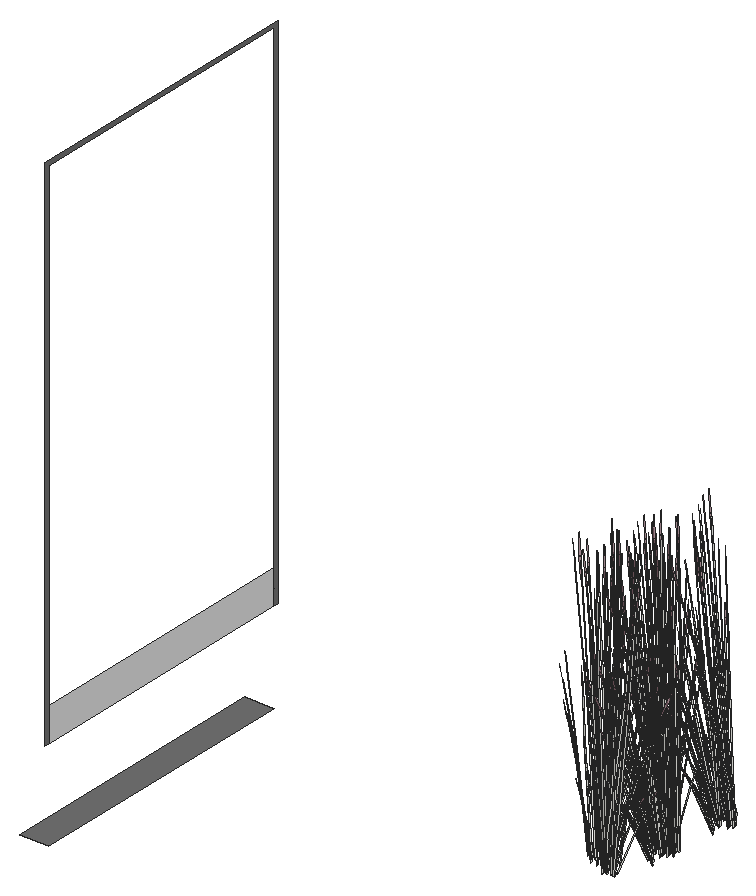
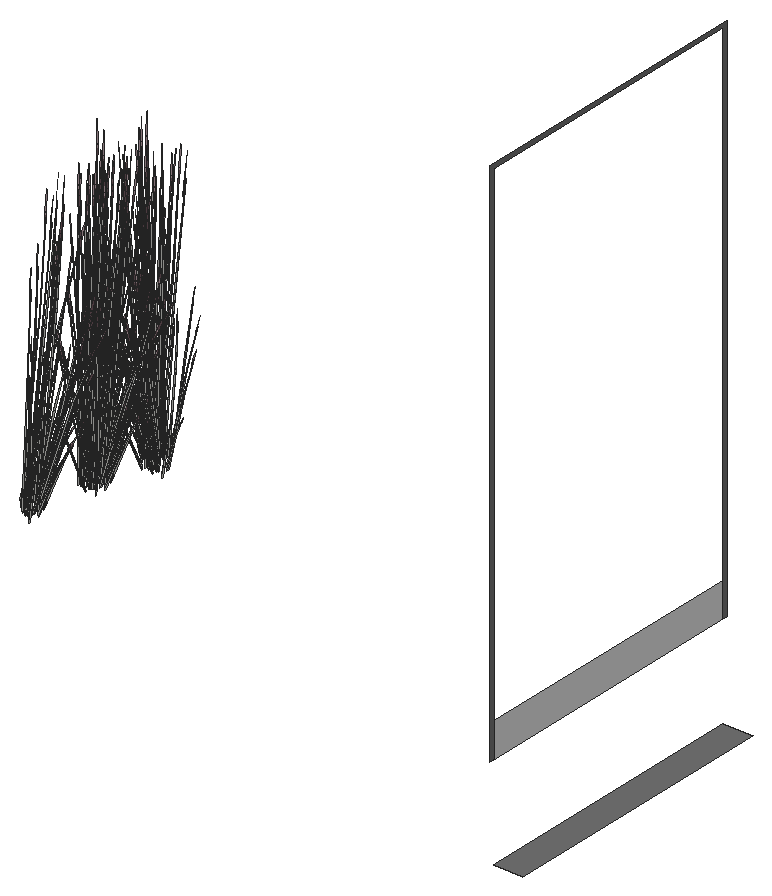
# SketchUp Ruby script. Lengths in inches.
U = 1.inch
M = Sketchup.active_model
def pt(a) = Geom::Point3d.new(a.map { |v| v * U })
def face(e, loops, mat)
  f = e.add_face(loops[0].map { |a| pt(a) })
  loops[1..].each { |l| e.add_face(l.map { |a| pt(a) }).erase! }
  f.material = f.back_material = mat if mat
  f
end
# faces: each face lists its corners as indices into pts; further lists are holes
def faces(e, pts, list, mat = nil) = list.each { |f| face(e, (f[0].is_a?(Array) ? f : [f]).map { |l| l.map { |i| pts[i] } }, mat) }
# xy, xz, yz: faces in a plane at the given z, y or x. An outline is a flat list of corners, or four numbers for a rectangle; further outlines are holes
def ring(l) = l.size == 4 ? [[l[0], l[1]], [l[2], l[1]], [l[2], l[3]], [l[0], l[3]]] : l.each_slice(2).to_a
def flat(e, list, mat, &to3) = list.each { |f| face(e, (f[0].is_a?(Array) ? f : [f]).map { |l| ring(l).map { |u, v| to3.(u, v) } }, mat) }
def xy(e, z, list, mat = nil) = flat(e, list, mat) { |x, y| [x, y, z] }
def xz(e, y, list, mat = nil) = flat(e, list, mat) { |x, z| [x, y, z] }
def yz(e, x, list, mat = nil) = flat(e, list, mat) { |y, z| [x, y, z] }
def lines(e, pts, list) = list.each { |a, b| e.add_line(pt(pts[a]), pt(pts[b])) }
# prism: a flat outline (further loops are holes) pulled along v
def prism(e, loops, v, mat = nil)
  f = face(e, loops, mat); d = Geom::Vector3d.new(v.map { |x| x * U })
  f.pushpull(f.normal.samedirection?(d) ? d.length : -d.length)
end
def box(e, o, s, mat = nil) = prism(e, [[o, [o[0] + s[0], o[1], o[2]], [o[0] + s[0], o[1] + s[1], o[2]], [o[0], o[1] + s[1], o[2]]]], [0, 0, s[2]], mat)
def at(x, y, z, deg = 0) = Geom::Transformation.translation(pt([x, y, z])) * Geom::Transformation.rotation(ORIGIN, Z_AXIS, deg.degrees)
def axes(o, x, y, z) = Geom::Transformation.new([*x, 0, *y, 0, *z, 0, *pt(o).to_a, 1])
def part(name) = M.definitions.add(name)
# library, detail: a bought-in or finely detailed component or shape, given as its bounding box
def library(name, o, s) = part(name).tap { |d| box(d.entities, o, s) }
def detail(e, o, s) = box(e.add_group.entities, o, s)
def put(e, d, t, mat = nil) = e.add_instance(d, t).tap { |i| i.material = mat if mat }
def group(e, t, mat = nil) = e.add_group.tap { |g| g.transformation = t; g.material = mat if mat }.entities
root = M.entities
M.materials.add("LightPink_Translucent").color = [144, 107, 117]
M.materials["LightPink_Translucent"].alpha = 0.75
M.materials.add("M01_Silver_Fog").color = [224, 224, 224]
M.materials.add("M06_Steel_Smoke").color = [114, 114, 114]
c1 = part("blade")
p = [[2.15,0.21,22],[0,0.17,0],[0.09,0.45,0],[2.18,0.31,22],[2.29,0.31,22],[0.38,0.45,0],
  [2.48,0.24,33],[2.49,0.24,33],[2.48,0.22,33]]
faces(c1.entities,p,[[0,1,2,3],[4,5,2,3],[6,3,4,7],[8,0,3,6]])
c2 = part("seeds")
p = [[0.3,-0.1,1.38],[-0.01,-0.03,1.59],[-0.01,-0.03,0.03],[0.14,-0.07,-0.07],[0.29,-0.03,3],[0.15,0.01,3.11]]
faces(c2.entities,p,[[0,1,2,3],[1,0,4,5]],"LightPink_Translucent")
c3 = part("blade with seeds")
put(c3.entities,c1,at(0,0,0))
put(c3.entities,c2,axes([2.4,0.25,30.99],[1.5799,-0.05474,1.17369],[-0.12525,1.92788,0.29478],[-0.07173,-0.02425,1.56792]))
xy(root,503,[[204,295,210,353]],"M06_Steel_Smoke")
yz(root,210,[[295,522,353,529]],"M01_Silver_Fog")
yz(root,210,[[294,522,295,522,295,629,353,629,353,522,354,522,354,630,294,630]],"M06_Steel_Smoke")
put(root,c3,axes([306.14,314.57,525.875],[0.17434,-0.11391,1.71376],[0.14677,0.52637,0.13857],[-0.27369,0.11897,0.73262]))
put(root,c3,axes([305.6,315.47,524.59],[0.17462,0.04421,1.43002],[0.11254,0.45156,-0.30754],[-0.23719,0.08453,0.61141]))
put(root,c3,axes([306.16,314.32,526.68],[-0.13612,0.48987,-0.51099],[-0.46669,-0.16791,-0.3958],[-0.1879,0.04492,0.97773]))
put(root,c3,axes([305.23,316.41,524.77],[0.2094,-0.24408,1.1486],[0.08263,0.38639,0.84392],[-0.15132,0.06919,0.25299]))
put(root,c3,axes([306.78,314.92,525.875],[0.1255,-0.16547,1.71376],[0.31687,0.44665,0.13857],[-0.21734,0.2034,0.73262]))
put(root,c3,axes([306.02,315.36,526.53],[-0.43736,0.07697,-0.35414],[-0.11549,-0.43998,0.4572],[-0.12533,0.11818,0.87481]))
put(root,c3,axes([305.79,316.66,523.49],[0.0674,0.0538,1.76342],[0.11428,0.49852,-0.26939],[-0.14937,0.10631,0.30037]))
put(root,c3,axes([306.6875,315.33,525.875],[0.09355,-0.18511,1.71376],[0.39247,0.38307,0.13857],[-0.17705,0.23875,0.73262]))
put(root,c3,axes([306.38,315.41,526.68],[0.12908,0.49174,-0.51099],[-0.48882,0.08602,-0.3958],[-0.14008,0.13208,0.97773]))
put(root,c3,axes([307.2,316.41,524.375],[-0.31414,0.53965,0],[-0.52557,-0.30095,-0.51607],[-0.1197,-0.06854,1.63711]))
put(root,c3,axes([306.63,317.19,524.59],[0.15856,-0.08496,1.43002],[0.39147,0.25616,-0.30754],[-0.11652,0.22165,0.61141]))
put(root,c3,axes([306.79,316.375,526.53],[-0.33997,0.28354,-0.35414],[-0.32182,-0.32376,0.4572],[-0.04897,0.1645,0.87481]))
put(root,c3,axes([308.53,315.53,524.06],[-0.33843,0.40479,-0.62353],[-0.42041,-0.36705,-0.16365],[-0.13561,0.10098,1.37633]))
put(root,c3,axes([310.75,324.63,525.875],[0.20841,-0.0122,1.71376],[-0.13825,0.52864,0.13857],[-0.297,-0.0327,0.73262]))
put(root,c3,axes([308.77,315.3,524.46],[-0.49063,-0.43346,-0.25192],[0.41285,-0.48673,0.5513],[-0.13212,0.05071,1.68216]))
put(root,c3,axes([307.02,316.08,527.34],[-0.01307,0.49815,-0.7886],[-0.55054,-0.03346,0.09517],[-0.0581,0.21104,1.11556]))
put(root,c3,axes([307.01,317.48,524.77],[-0.013,-0.32022,1.1486],[0.32493,0.22839,0.84392],[-0.0639,0.15263,0.25299]))
put(root,c3,axes([308.52,315.21,524.21],[-0.54562,0.03324,-0.44739],[-0.04934,-0.55185,0.21531],[-0.09768,0.05593,1.43643]))
put(root,c3,axes([307.48,316.13,524.48],[0.47024,0.26927,0.49651],[-0.28107,0.48284,0],[-0.1071,-0.06133,1.57504]))
put(root,c3,axes([310.84,325.56,525.875],[0.17434,-0.11391,1.71376],[0.14677,0.52637,0.13857],[-0.27369,0.11897,0.73262]))
put(root,c3,axes([306.84,316.78,525.36],[0.01104,-0.27801,1.54345],[0.49652,0.14685,0.21329],[-0.04302,0.2963,0.72882]))
put(root,c3,axes([310.29,326.46,524.59],[0.17462,0.04421,1.43002],[0.11254,0.45156,-0.30754],[-0.23719,0.08453,0.61141]))
put(root,c3,axes([309.09,316.63,524.02],[-0.47024,0.26927,-0.49651],[-0.28107,-0.48284,0],[-0.1071,0.06133,1.57504]))
put(root,c3,axes([309.12,316.49,524.19],[-0.31023,-0.54153,-0.05142],[0.52557,-0.30095,0.51607],[-0.12951,0.05156,1.6363]))
put(root,c3,axes([311.84,325.01,525.34],[0.14282,-0.0779,1.77064],[0.04925,0.54394,0.13857],[-0.30935,0.07218,0.63284]))
put(root,c3,axes([307.13,316.24,527],[0.35968,0.36185,-0.5672],[-0.37996,0.3169,-0.43934],[-0.05473,0.18385,1.08528]))
put(root,c3,axes([308.98,316.42,524.03],[-0.46876,-0.13325,-0.30978],[0.11803,-0.46926,0.30978],[-0.0945,0.05411,1.38974]))
put(root,c3,axes([309.25,314.41,524.84],[-0.01373,-0.50706,1.41272],[0.62119,0.13144,0.59816],[-0.14692,0.27746,1.3335]))
put(root,c3,axes([311.375,324.14,526.98],[-0.50227,-0.01297,-0.71045],[0.03373,-0.54602,0.08574],[-0.21278,-0.05762,1.00501]))
put(root,c3,axes([310.97,324.27,524.59],[0.0981,0.14994,1.43002],[-0.22605,0.40756,-0.30754],[-0.23211,-0.09741,0.61141]))
put(root,c3,axes([306.74,316.79,524.82],[0.45645,-0.09537,0.06507],[0.10494,0.38421,-0.86304],[-0.02894,0.19449,0.7736]))
put(root,c3,axes([308.9,315.06,524.67],[0.05855,0.61451,-0.29095],[-0.60981,0.03716,-0.50002],[-0.10738,0.08185,1.59708]))
put(root,c3,axes([310.57,325.08,526.53],[-0.41757,-0.15024,-0.35414],[0.12179,-0.4383,0.4572],[-0.16812,0.04019,0.87481]))
put(root,c3,axes([311.14,323.78,525.875],[0.18664,0.09279,1.71376],[-0.38624,0.38925,0.13857],[-0.24072,-0.1756,0.73262]))
put(root,c3,axes([307.54,315.72,525.875],[-0.0123,-0.2067,1.71376],[0.53301,0.13712,0.13857],[-0.03297,0.29456,0.73262]))
put(root,c3,axes([310.85,325.31,526.68],[-0.13612,0.48987,-0.51099],[-0.46669,-0.16791,-0.3958],[-0.1879,0.04492,0.97773]))
put(root,c3,axes([311.21,324.25,526.68],[-0.36484,0.35674,-0.51099],[-0.31952,-0.37685,-0.3958],[-0.18537,-0.05428,0.97773]))
put(root,c3,axes([310.62,325.28,523.49],[0.01274,0.08487,1.76342],[-0.25688,0.44323,-0.26939],[-0.18246,-0.02234,0.30037]))
put(root,c3,axes([309.93,327.4,524.77],[0.2094,-0.24408,1.1486],[0.08263,0.38639,0.84392],[-0.15132,0.06919,0.25299]))
put(root,c3,axes([308.35,315.94,524.2],[-0.50654,-0.24178,0],[0.24378,-0.50239,0],[0,0,1.62707]))
put(root,c3,axes([309.52,316.55,524.375],[0.31414,0.53965,0],[-0.52557,0.30095,-0.51607],[-0.1197,0.06854,1.63711]))
put(root,c3,axes([311.07,323.91,526.53],[-0.28589,-0.33718,-0.35414],[0.32644,-0.31919,0.4572],[-0.16586,-0.04856,0.87481]))
put(root,c3,axes([311.48,325.91,525.875],[0.1255,-0.16547,1.71376],[0.31687,0.44665,0.13857],[-0.21734,0.2034,0.73262]))
put(root,c3,axes([310.72,326.35,526.53],[-0.43736,0.07697,-0.35414],[-0.11549,-0.43998,0.4572],[-0.12533,0.11818,0.87481]))
put(root,c3,axes([310.48,327.65,523.49],[0.0674,0.0538,1.76342],[0.11428,0.49852,-0.26939],[-0.14937,0.10631,0.30037]))
put(root,c3,axes([309.01,315.18,524.62],[0.37121,0.32357,0.1448],[-0.30963,0.36505,-0.41347],[-0.08619,0.04935,1.26744]))
put(root,c3,axes([310.39,324.72,524.77],[0.32078,-0.03854,1.1486],[-0.20348,0.33954,0.84392],[-0.15852,-0.05093,0.25299]))
put(root,c3,axes([309,314.94,524.72],[0.54562,-0.03324,0.44739],[0.04934,0.55185,-0.21531],[-0.09768,0.05593,1.43643]))
put(root,c3,axes([309.14,316.21,524.33],[0.62903,0.17504,0.30756],[-0.15737,0.62568,-0.36492],[-0.10411,0.07831,1.64885]))
put(root,c3,axes([309.41,316.17,524.48],[0.47024,-0.26927,0.49651],[0.28107,0.48284,0],[-0.1071,0.06133,1.57504]))
put(root,c3,axes([307.87,316.71,523.49],[0.08132,-0.0293,1.76342],[0.48914,0.1613,-0.26939],[0.0143,0.18179,0.30037]))
put(root,c3,axes([311.38,326.32,525.875],[0.09355,-0.18511,1.71376],[0.39247,0.38307,0.13857],[-0.17705,0.23875,0.73262]))
put(root,c3,axes([307.97,316.875,526.53],[-0.15148,0.41415,-0.35414],[-0.44193,-0.12079,0.4572],[0.04052,0.16674,0.87481]))
put(root,c3,axes([313.57,337.98,525.875],[0.20841,-0.0122,1.71376],[-0.13825,0.52864,0.13857],[-0.297,-0.0327,0.73262]))
put(root,c3,axes([311.08,326.4,526.68],[0.12908,0.49174,-0.51099],[-0.48882,0.08602,-0.3958],[-0.14008,0.13208,0.97773]))
put(root,c3,axes([309.12,314.82,524.21],[-0.24378,0.48527,-0.44739],[-0.50654,-0.23354,0.21531],[0,0.11186,1.43643]))
put(root,c3,axes([312.3,326.05,524.06],[-0.52267,-0.08829,-0.62353],[0.11029,-0.54463,-0.16365],[-0.15598,-0.06599,1.37633]))
put(root,c3,axes([312.25,323.5,526.98],[-0.42844,-0.2603,-0.71045],[0.30448,-0.45614,0.08574],[-0.15523,-0.15542,1.00501]))
put(root,c3,axes([312.05,323.51,526.68],[-0.4958,0.12802,-0.51099],[-0.08673,-0.48481,-0.3958],[-0.13317,-0.13893,0.97773]))
put(root,c3,axes([309.04,314.54,524.29],[0,0.62282,-0.05637],[-0.62828,0,0],[0,0.01957,1.79368]))
put(root,c3,axes([313.66,338.91,525.875],[0.17434,-0.11391,1.71376],[0.14677,0.52637,0.13857],[-0.27369,0.11897,0.73262]))
put(root,c3,axes([311.61,327.08,524.02],[-0.47024,-0.26927,-0.49651],[0.28107,-0.48284,0],[-0.1071,-0.06133,1.57504]))
put(root,c3,axes([308.74,315.75,524.29],[0.21845,0.61869,-0.06012],[-0.62418,0.21679,0],[0.00763,0.02161,1.72173]))
put(root,c3,axes([311.41,323.07,523.49],[-0.04867,0.07094,1.76342],[-0.49185,0.15296,-0.26939],[-0.11882,-0.13915,0.30037]))
put(root,c3,axes([313.12,339.8125,524.59],[0.17462,0.04421,1.43002],[0.11254,0.45156,-0.30754],[-0.23719,0.08453,0.61141]))
put(root,c3,axes([311.9,327.4,524.375],[-0.31414,0.53965,0],[-0.52557,-0.30095,-0.51607],[-0.1197,-0.06854,1.63711]))
put(root,c3,axes([314.66,338.36,525.34],[0.14282,-0.0779,1.77064],[0.04925,0.54394,0.13857],[-0.30935,0.07218,0.63284]))
put(root,c3,axes([308.02,316.5,526.98],[0.23981,0.43789,-0.71045],[-0.49365,0.24404,0.08574],[0.05608,0.21158,1.00501]))
put(root,c3,axes([310.54,314.9375,524.2],[-0.62797,-0.00431,-0.04976],[0,-0.6019,0.49943],[-0.01973,0.13702,1.58352]))
put(root,c3,axes([311.33,328.18,524.59],[0.15856,-0.08496,1.43002],[0.39147,0.25616,-0.30754],[-0.11652,0.22165,0.61141]))
put(root,c3,axes([311.1,323.34,524.13],[-0.14494,0.43975,-0.03893],[-0.4461,-0.13527,-0.17649],[-0.06773,-0.07192,0.58215]))
put(root,c3,axes([309.13,314.27,524.72],[0.24378,-0.48527,0.44739],[0.50654,0.23354,-0.21531],[0,0.11186,1.43643]))
put(root,c3,axes([308.92,315.95,524.2],[0.50654,0.24178,0],[-0.24378,0.50239,0],[0,0,1.74954]))
put(root,c3,axes([314.2,337.49,526.98],[-0.50227,-0.01297,-0.71045],[0.03373,-0.54602,0.08574],[-0.21278,-0.05762,1.00501]))
put(root,c3,axes([313.79,337.625,524.59],[0.0981,0.14994,1.43002],[-0.22605,0.40756,-0.30754],[-0.23211,-0.09741,0.61141]))
put(root,c3,axes([308.2,316.59,526.68],[0.49392,0.135,-0.51099],[-0.1693,0.46287,-0.3958],[0.04529,0.18636,0.97773]))
put(root,c3,axes([311.77,322.79,524.59],[-0.03043,0.17617,1.43002],[-0.4448,0.14748,-0.30754],[-0.10397,-0.22771,0.61141]))
put(root,c3,axes([313.39,338.4375,526.53],[-0.41757,-0.15024,-0.35414],[0.12179,-0.4383,0.4572],[-0.16812,0.04019,0.87481]))
put(root,c3,axes([313.97,337.13,525.875],[0.18664,0.09279,1.71376],[-0.38624,0.38925,0.13857],[-0.24072,-0.1756,0.73262]))
put(root,c3,axes([311.91,323.24,525.875],[0.11485,0.17291,1.71376],[-0.53072,0.14557,0.13857],[-0.11995,-0.27145,0.73262]))
put(root,c3,axes([312.89,326.125,524.67],[-0.5073,0.35754,-0.29095],[-0.33735,-0.5052,-0.50002],[-0.12516,-0.05131,1.59708]))
put(root,c3,axes([310.41,315.03,524.03],[-0.35073,0.33601,-0.30978],[-0.35073,-0.33601,0.30978],[0,0.10823,1.38974]))
put(root,c3,axes([312.1,323.15,526.53],[-0.0776,-0.43378,-0.35414],[0.44361,-0.11454,0.4572],[-0.11915,-0.12431,0.87481]))
put(root,c3,axes([309.41,314.96,524.09],[0.18424,0.49308,-0.69212],[-0.53071,0.17758,-0.18165],[0.02036,0.16697,1.52773]))
put(root,c3,axes([310.86,325.35,524.375],[-0.62828,0,0],[0,-0.6019,-0.51607],[0,-0.13709,1.63711]))
put(root,c3,axes([311.74,326.875,524.03],[-0.11803,-0.46926,-0.30978],[0.46876,-0.13325,0.30978],[-0.0945,-0.05411,1.38974]))
put(root,c3,axes([313.68,338.66,526.68],[-0.13612,0.48987,-0.51099],[-0.46669,-0.16791,-0.3958],[-0.1879,0.04492,0.97773]))
put(root,c3,axes([311.49,327.37,526.53],[-0.33997,0.28354,-0.35414],[-0.32182,-0.32376,0.4572],[-0.04897,0.1645,0.87481]))
put(root,c3,axes([309.34,314.38,524.62],[0.46814,-0.15705,0.1448],[0.16394,0.44848,-0.41347],[0,0.0987,1.26744]))
put(root,c3,axes([314.03,337.6,526.68],[-0.36484,0.35674,-0.51099],[-0.31952,-0.37685,-0.3958],[-0.18537,-0.05428,0.97773]))
put(root,c3,axes([313.44,338.63,523.49],[0.01274,0.08487,1.76342],[-0.25688,0.44323,-0.26939],[-0.18246,-0.02234,0.30037]))
put(root,c3,axes([313.23,326.52,524.06],[-0.33843,0.40479,-0.62353],[-0.42041,-0.36705,-0.16365],[-0.13561,0.10098,1.37633]))
put(root,c3,axes([309.18,314.41,524.67],[0.56585,0.25696,-0.29095],[-0.27246,0.54236,-0.50002],[0.01778,0.13316,1.59708]))
put(root,c3,axes([311.35,325.1875,524.33],[-0.46736,0.45277,0.30756],[-0.46764,-0.44801,-0.36492],[-0.01632,-0.12858,1.64885]))
put(root,c3,axes([312.75,340.76,524.77],[0.2094,-0.24408,1.1486],[0.08263,0.38639,0.84392],[-0.15132,0.06919,0.25299]))
put(root,c3,axes([313.27,326.44,525.33],[0.4342,0.21716,1.51261],[-0.42537,0.46784,0.59816],[-0.19053,-0.27728,1.26806]))
put(root,c3,axes([311.62,322.5,524.77],[0.2621,0.18744,1.1486],[-0.38171,0.11267,0.84392],[-0.08167,-0.14405,0.25299]))
put(root,c3,axes([313.46,326.29,524.46],[-0.49063,-0.43346,-0.25192],[0.41285,-0.48673,0.5513],[-0.13212,0.05071,1.68216]))
put(root,c3,axes([312.57,325.87,524.21],[-0.30184,-0.45202,-0.44739],[0.45719,-0.31831,0.21531],[-0.09768,-0.05593,1.43643]))
put(root,c3,axes([310.41,314.54,524.48],[0,-0.53854,0.49651],[0.56215,0,0],[0,0.12266,1.57504]))
put(root,c3,axes([311.72,327.07,527.34],[-0.01307,0.49815,-0.7886],[-0.55054,-0.03346,0.09517],[-0.0581,0.21104,1.11556]))
put(root,c3,axes([310.65,315.04,524.02],[0,0.53854,-0.49651],[-0.56215,0,0],[0,0.12266,1.57504]))
put(root,c3,axes([313.89,337.27,526.53],[-0.28589,-0.33718,-0.35414],[0.32644,-0.31919,0.4572],[-0.16586,-0.04856,0.87481]))
put(root,c3,axes([308.48,315.64,525.875],[-0.11485,-0.17291,1.71376],[0.53072,-0.14557,0.13857],[0.11995,0.27145,0.73262]))
put(root,c3,axes([311.71,328.47,524.77],[-0.013,-0.32022,1.1486],[0.32493,0.22839,0.84392],[-0.0639,0.15263,0.25299]))
put(root,c3,axes([314.3,339.27,525.875],[0.1255,-0.16547,1.71376],[0.31687,0.44665,0.13857],[-0.21734,0.2034,0.73262]))
put(root,c3,axes([313.54,339.7,526.53],[-0.43736,0.07697,-0.35414],[-0.11549,-0.43998,0.4572],[-0.12533,0.11818,0.87481]))
put(root,c3,axes([313.21,326.2,524.21],[-0.54562,0.03324,-0.44739],[-0.04934,-0.55185,0.21531],[-0.09768,0.05593,1.43643]))
put(root,c3,axes([313.3,341.01,523.49],[0.0674,0.0538,1.76342],[0.11428,0.49852,-0.26939],[-0.14937,0.10631,0.30037]))
put(root,c3,axes([313.21,338.08,524.77],[0.32078,-0.03854,1.1486],[-0.20348,0.33954,0.84392],[-0.15852,-0.05093,0.25299]))
put(root,c3,axes([312.17,327.12,524.48],[0.47024,0.26927,0.49651],[-0.28107,0.48284,0],[-0.1071,-0.06133,1.57504]))
put(root,c3,axes([311.53,327.77,525.36],[0.01104,-0.27801,1.54345],[0.49652,0.14685,0.21329],[-0.04302,0.2963,0.72882]))
put(root,c3,axes([312.61,326.13,524.4375],[0.13317,-0.63814,-0.23429],[0.63143,0.11124,0.51271],[-0.11033,-0.08813,1.5644]))
put(root,c3,axes([312.84,326.28,524.62],[-0.09693,0.48062,0.1448],[-0.47357,-0.08343,-0.41347],[-0.08619,-0.04935,1.26744]))
put(root,c3,axes([313.79,327.62,524.02],[-0.47024,0.26927,-0.49651],[-0.28107,-0.48284,0],[-0.1071,0.06133,1.57504]))
put(root,c3,axes([311,324.9375,524.02],[0,-0.53854,-0.49651],[0.56215,0,0],[0,-0.12266,1.57504]))
put(root,c3,axes([311.24,325.4375,524.48],[0,0.53854,0.49651],[-0.56215,0,0],[0,-0.12266,1.57504]))
put(root,c3,axes([313.82,327.48,524.19],[-0.31023,-0.54153,-0.05142],[0.52557,-0.30095,0.51607],[-0.12951,0.05156,1.6363]))
put(root,c3,axes([309.08,314.1,524.21],[0.30184,0.45202,-0.44739],[-0.45719,0.31831,0.21531],[0.09768,0.05593,1.43643]))
put(root,c3,axes([314.2,339.68,525.875],[0.09355,-0.18511,1.71376],[0.39247,0.38307,0.13857],[-0.17705,0.23875,0.73262]))
put(root,c3,axes([311.83,327.23,527],[0.35968,0.36185,-0.5672],[-0.37996,0.3169,-0.43934],[-0.05473,0.18385,1.08528]))
put(root,c3,axes([313.68,327.41,524.03],[-0.46876,-0.13325,-0.30978],[0.11803,-0.46926,0.30978],[-0.0945,0.05411,1.38974]))
put(root,c3,axes([312.47,325.5625,524.67],[-0.56585,-0.25696,-0.29095],[0.27246,-0.54236,-0.50002],[-0.01778,-0.13316,1.59708]))
put(root,c3,axes([309.9375,316.15,524.77],[-0.2829,-0.15485,1.1486],[0.36529,-0.15734,0.84392],[0.09853,0.13328,0.25299]))
put(root,c3,axes([313.95,325.4,524.84],[-0.01373,-0.50706,1.41272],[0.62119,0.13144,0.59816],[-0.14692,0.27746,1.3335]))
put(root,c3,axes([308.93,315.99,524.59],[0.00887,-0.17852,1.43002],[0.42372,-0.19941,-0.30754],[0.1308,0.21367,0.61141]))
put(root,c3,axes([313.9,339.75,526.68],[0.12908,0.49174,-0.51099],[-0.48882,0.08602,-0.3958],[-0.14008,0.13208,0.97773]))
put(root,c3,axes([315.12,339.4,524.06],[-0.52267,-0.08829,-0.62353],[0.11029,-0.54463,-0.16365],[-0.15598,-0.06599,1.37633]))
put(root,c3,axes([311.4375,327.78,524.82],[0.45645,-0.09537,0.06507],[0.10494,0.38421,-0.86304],[-0.02894,0.19449,0.7736]))
put(root,c3,axes([313.6,326.05,524.67],[0.05855,0.61451,-0.29095],[-0.60981,0.03716,-0.50002],[-0.10738,0.08185,1.59708]))
put(root,c3,axes([312.22,325.02,524.1],[-0.20635,-0.55225,-0.69835],[0.59439,-0.19889,-0.18329],[-0.02281,-0.18701,1.54149]))
put(root,c3,axes([313.15,323.28,526.68],[-0.49392,-0.135,-0.51099],[0.1693,-0.46287,-0.3958],[-0.04529,-0.18636,0.97773]))
put(root,c3,axes([310.79,314.63,524.375],[0.62828,0,0],[0,0.6019,-0.51607],[0,0.13709,1.63711]))
put(root,c3,axes([315.07,336.85,526.98],[-0.42844,-0.2603,-0.71045],[0.30448,-0.45614,0.08574],[-0.15523,-0.15542,1.00501]))
put(root,c3,axes([314.87,336.86,526.68],[-0.4958,0.12802,-0.51099],[-0.08673,-0.48481,-0.3958],[-0.13317,-0.13893,0.97773]))
put(root,c3,axes([312.24,326.71,525.875],[-0.0123,-0.2067,1.71376],[0.53301,0.13712,0.13857],[-0.03297,0.29456,0.73262]))
put(root,c3,axes([311.24,324.95,524.03],[0.35073,-0.33601,-0.30978],[0.35073,0.33601,0.30978],[0,-0.10823,1.38974]))
put(root,c3,axes([312.83,322.78,524.13],[-0.34721,0.30895,-0.03893],[-0.31814,-0.33837,-0.17649],[-0.0224,-0.09588,0.58215]))
put(root,c3,axes([309.98,316.86,524.67],[-0.3222,-0.01689,1.0506],[0.21278,-0.35872,0.58006],[0.12729,0.12745,0.8241]))
put(root,c3,axes([314.44,340.43,524.02],[-0.47024,-0.26927,-0.49651],[0.28107,-0.48284,0],[-0.1071,-0.06133,1.57504]))
put(root,c3,axes([312.6875,325.82,524.36],[0.63506,0.11347,0.45755],[-0.12924,0.64083,0.17955],[-0.09281,-0.06188,1.58856]))
put(root,c3,axes([314.23,336.42,523.49],[-0.04867,0.07094,1.76342],[-0.49185,0.15296,-0.26939],[-0.11882,-0.13915,0.30037]))
put(root,c3,axes([314.72,340.76,524.375],[-0.31414,0.53965,0],[-0.52557,-0.30095,-0.51607],[-0.1197,-0.06854,1.63711]))
put(root,c3,axes([312.52,325.71,524.72],[-0.24378,0.48527,0.44739],[-0.50654,-0.23354,-0.21531],[0,-0.11186,1.43643]))
put(root,c3,axes([313.33,323.37,526.98],[-0.23981,-0.43789,-0.71045],[0.49365,-0.24404,0.08574],[-0.05608,-0.21158,1.00501]))
put(root,c3,axes([312.35,326.85,524.47],[0.53992,-0.14294,0.17642],[0.13332,0.53195,0.35086],[-0.04815,-0.07751,1.60407]))
put(root,c3,axes([313.04,326.93,524.2],[-0.50654,-0.24178,0],[0.24378,-0.50239,0],[0,0,1.62707]))
put(root,c3,axes([314.21,327.54,524.375],[0.31414,0.53965,0],[-0.52557,0.30095,-0.51607],[-0.1197,0.06854,1.63711]))
put(root,c3,axes([313.92,336.69,524.13],[-0.14494,0.43975,-0.03893],[-0.4461,-0.13527,-0.17649],[-0.06773,-0.07192,0.58215]))
put(root,c3,axes([309.3,316.37,526.68],[0.4958,-0.12802,-0.51099],[0.08673,0.48481,-0.3958],[0.13317,0.13893,0.97773]))
put(root,c3,axes([314.59,336.14,524.59],[-0.03043,0.17617,1.43002],[-0.4448,0.14748,-0.30754],[-0.10397,-0.22771,0.61141]))
put(root,c3,axes([313.95,326.88,524.47],[0.14515,-0.53522,0.17642],[0.53115,0.15146,0.35086],[-0.09175,0.00261,1.60407]))
put(root,c3,axes([313.71,326.17,524.62],[0.37121,0.32357,0.1448],[-0.30963,0.36505,-0.41347],[-0.08619,0.04935,1.26744]))
put(root,c3,axes([314.74,336.6,525.875],[0.11485,0.17291,1.71376],[-0.53072,0.14557,0.13857],[-0.11995,-0.27145,0.73262]))
put(root,c3,axes([315.71,339.48,524.67],[-0.5073,0.35754,-0.29095],[-0.33735,-0.5052,-0.50002],[-0.12516,-0.05131,1.59708]))
put(root,c3,axes([310.02,316.73,523.49],[0.03661,-0.07775,1.76342],[0.46087,-0.22898,-0.26939],[0.13972,0.11851,0.30037]))
put(root,c3,axes([313.58,325.77,524.3],[-0.46736,-0.46353,-0.06131],[0.46764,-0.46381,0],[-0.01632,-0.01619,1.75571]))
put(root,c3,axes([313.7,325.93,524.72],[0.54562,-0.03324,0.44739],[0.04934,0.55185,-0.21531],[-0.09768,0.05593,1.43643]))
put(root,c3,axes([314.92,336.5,526.53],[-0.0776,-0.43378,-0.35414],[0.44361,-0.11454,0.4572],[-0.11915,-0.12431,0.87481]))
put(root,c3,axes([313.68,338.7,524.375],[-0.62828,0,0],[0,-0.6019,-0.51607],[0,-0.13709,1.63711]))
put(root,c3,axes([314.57,340.23,524.03],[-0.11803,-0.46926,-0.30978],[0.46876,-0.13325,0.30978],[-0.0945,-0.05411,1.38974]))
put(root,c3,axes([311.125,316.01,525.93],[-0.09617,-0.45271,-0.03492],[0.45453,-0.10408,-0.15832],[0.09492,0.0287,0.52218]))
put(root,c3,axes([313.83,327.2,524.33],[0.62903,0.17504,0.30756],[-0.15737,0.62568,-0.36492],[-0.10411,0.07831,1.64885]))
put(root,c3,axes([312.91,322.4,523.49],[-0.08428,0.0194,1.76342],[-0.46606,-0.21841,-0.26939],[0.00782,-0.18218,0.30037]))
put(root,c3,axes([314.1,327.16,524.48],[0.47024,-0.26927,0.49651],[0.28107,0.48284,0],[-0.1071,0.06133,1.57504]))
put(root,c3,axes([313.375,323,526.53],[0.15148,-0.41415,-0.35414],[0.44193,0.12079,0.4572],[-0.04052,-0.16674,0.87481]))
put(root,c3,axes([312.63,325.23,524.36],[0.21845,0.6022,0.45755],[-0.62418,0.20941,0.17955],[0.00763,-0.11065,1.58856]))
put(root,c3,axes([312.53,325.16,524.21],[0.24378,-0.48527,-0.44739],[0.50654,0.23354,0.21531],[0,-0.11186,1.43643]))
put(root,c3,axes([313.16,326.72,524.2],[-0.16394,-0.4643,0],[0.46814,-0.1626,0],[0,0,1.54371]))
put(root,c3,axes([316.05,339.87,524.06],[-0.33843,0.40479,-0.62353],[-0.42041,-0.36705,-0.16365],[-0.13561,0.10098,1.37633]))
put(root,c3,axes([312.5625,327.7,523.49],[0.08132,-0.0293,1.76342],[0.48914,0.1613,-0.26939],[0.0143,0.18179,0.30037]))
put(root,c3,axes([312.67,327.87,526.53],[-0.15148,0.41415,-0.35414],[-0.44193,-0.12079,0.4572],[0.04052,0.16674,0.87481]))
put(root,c3,axes([314.17,338.54,524.33],[-0.46736,0.45277,0.30756],[-0.46764,-0.44801,-0.36492],[-0.01632,-0.12858,1.64885]))
put(root,c3,axes([316.09,339.79,525.33],[0.4342,0.21716,1.51261],[-0.42537,0.46784,0.59816],[-0.19053,-0.27728,1.26806]))
put(root,c3,axes([314.4375,335.85,524.77],[0.2621,0.18744,1.1486],[-0.38171,0.11267,0.84392],[-0.08167,-0.14405,0.25299]))
put(root,c3,axes([316.28,339.64,524.46],[-0.49063,-0.43346,-0.25192],[0.41285,-0.48673,0.5513],[-0.13212,0.05071,1.68216]))
put(root,c3,axes([315.39,339.23,524.21],[-0.30184,-0.45202,-0.44739],[0.45719,-0.31831,0.21531],[-0.09768,-0.05593,1.43643]))
put(root,c3,axes([313.82,325.81,524.21],[-0.24378,0.48527,-0.44739],[-0.50654,-0.23354,0.21531],[0,0.11186,1.43643]))
put(root,c3,axes([309.25,315.1,525.875],[-0.18664,-0.09279,1.71376],[0.38624,-0.38925,0.13857],[0.24072,0.1756,0.73262]))
put(root,c3,axes([316.04,339.55,524.21],[-0.54562,0.03324,-0.44739],[-0.04934,-0.55185,0.21531],[-0.09768,0.05593,1.43643]))
put(root,c3,axes([314.78,325.51,524.47],[-0.39477,-0.39228,0.17642],[0.39783,-0.38049,0.35086],[-0.0436,0.08011,1.60407]))
put(root,c3,axes([313.42,325.29,524.21],[0,-0.62313,0],[0.62828,0,0],[0,0,1.79456]))
